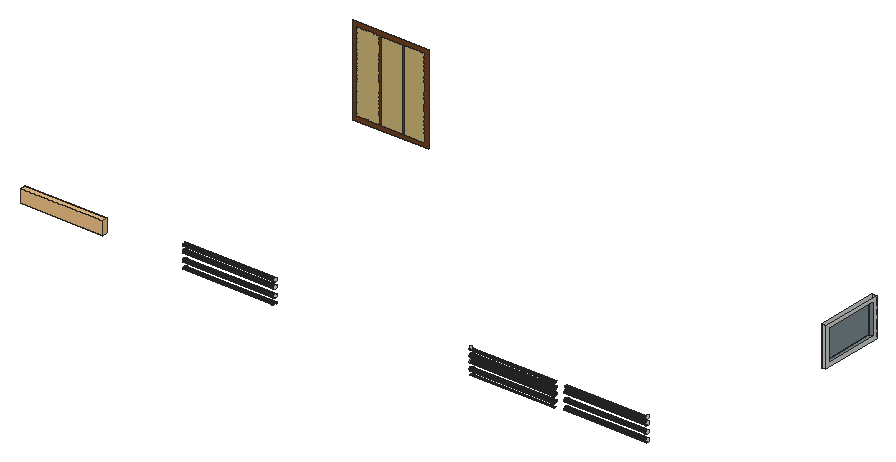
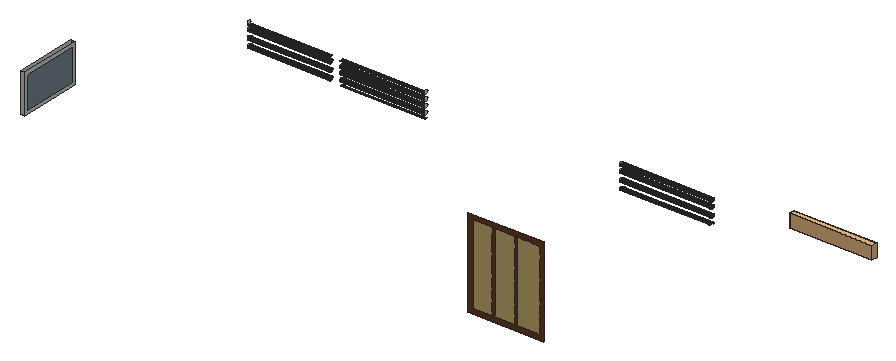
# SketchUp Ruby script. Lengths in inches.
U = 1.inch
M = Sketchup.active_model
def pt(a) = Geom::Point3d.new(a.map { |v| v * U })
def face(e, loops, mat)
  f = e.add_face(loops[0].map { |a| pt(a) })
  loops[1..].each { |l| e.add_face(l.map { |a| pt(a) }).erase! }
  f.material = f.back_material = mat if mat
  f
end
# faces: each face lists its corners as indices into pts; further lists are holes
def faces(e, pts, list, mat = nil) = list.each { |f| face(e, (f[0].is_a?(Array) ? f : [f]).map { |l| l.map { |i| pts[i] } }, mat) }
# xy, xz, yz: faces in a plane at the given z, y or x. An outline is a flat list of corners, or four numbers for a rectangle; further outlines are holes
def ring(l) = l.size == 4 ? [[l[0], l[1]], [l[2], l[1]], [l[2], l[3]], [l[0], l[3]]] : l.each_slice(2).to_a
def flat(e, list, mat, &to3) = list.each { |f| face(e, (f[0].is_a?(Array) ? f : [f]).map { |l| ring(l).map { |u, v| to3.(u, v) } }, mat) }
def xy(e, z, list, mat = nil) = flat(e, list, mat) { |x, y| [x, y, z] }
def xz(e, y, list, mat = nil) = flat(e, list, mat) { |x, z| [x, y, z] }
def yz(e, x, list, mat = nil) = flat(e, list, mat) { |y, z| [x, y, z] }
def lines(e, pts, list) = list.each { |a, b| e.add_line(pt(pts[a]), pt(pts[b])) }
# prism: a flat outline (further loops are holes) pulled along v
def prism(e, loops, v, mat = nil)
  f = face(e, loops, mat); d = Geom::Vector3d.new(v.map { |x| x * U })
  f.pushpull(f.normal.samedirection?(d) ? d.length : -d.length)
end
def box(e, o, s, mat = nil) = prism(e, [[o, [o[0] + s[0], o[1], o[2]], [o[0] + s[0], o[1] + s[1], o[2]], [o[0], o[1] + s[1], o[2]]]], [0, 0, s[2]], mat)
def at(x, y, z, deg = 0) = Geom::Transformation.translation(pt([x, y, z])) * Geom::Transformation.rotation(ORIGIN, Z_AXIS, deg.degrees)
def axes(o, x, y, z) = Geom::Transformation.new([*x, 0, *y, 0, *z, 0, *pt(o).to_a, 1])
def part(name) = M.definitions.add(name)
# library, detail: a bought-in or finely detailed component or shape, given as its bounding box
def library(name, o, s) = part(name).tap { |d| box(d.entities, o, s) }
def detail(e, o, s) = box(e.add_group.entities, o, s)
def put(e, d, t, mat = nil) = e.add_instance(d, t).tap { |i| i.material = mat if mat }
def group(e, t, mat = nil) = e.add_group.tap { |g| g.transformation = t; g.material = mat if mat }.entities
root = M.entities
M.materials.add("[Basic Tile]").color = [203, 206, 202]
M.materials.add("[Color M07]").color = [58, 58, 58]
M.materials.add("[Formica Speckled Grey]").color = [120, 135, 142]
M.materials.add("[Window Covering 02]").color = [199, 178, 115]
M.materials.add("[Wood Veneer 01]1").color = [109, 63, 33]
c1 = library("Housedekho",[1.1875,0,0],[76.76,10.33,12])
xy(root,109.0625,[[1639.03,679.86,1649.41,818.6]],"[Basic Tile]")
xy(root,117.18,[[1639.03,687.97,1649.41,810.49]],"[Formica Speckled Grey]")
xz(root,679.86,[[1639.03,109.0625,1649.41,194.8125]],"[Basic Tile]")
xz(root,687.97,[[1639.03,117.18,1649.41,186.7]],"[Formica Speckled Grey]")
xz(root,810.49,[[1639.03,117.18,1649.41,186.7]],"[Formica Speckled Grey]")
xz(root,818.6,[[1639.03,109.0625,1649.41,194.8125]],"[Basic Tile]")
xz(root,868.79,[[457.96,110.125,505.09,287.57],[513.29,110.125,556.28,287.57],[564.47,110.125,606.03,287.57]],"[Window Covering 02]")
xz(root,868.79,[[[448.22,100.38,615.78,297.32],[457.96,110.125,606.03,287.57]],[505.09,110.125,513.29,287.57],[556.28,110.125,564.47,287.57]],"[Wood Veneer 01]1")
yz(root,716.4,[[319.3,81.86,320.31,82,321.24,82.38,322.04,83,322.66,83.8,323.05,84.74,323.18,85.74,323.05,86.74,322.66,87.68,322.04,88.48,321.24,89.09,320.31,89.48,319.3,89.61,318.3,89.48,317.37,89.09,316.56,88.48,315.95,87.68,315.5625,86.74,315.43,85.74,315.5625,84.74,315.95,83.8,316.56,83,317.37,82.38,318.3,82],[319.3,99.55,320.31,99.68,321.24,100.07,322.04,100.6875,322.66,101.49,323.05,102.42,323.18,103.43,323.05,104.43,322.66,105.36,322.04,106.17,321.24,106.78,320.31,107.17,319.3,107.3,318.3,107.17,317.37,106.78,316.56,106.17,315.95,105.36,315.5625,104.43,315.43,103.43,315.5625,102.42,315.95,101.49,316.56,100.6875,317.37,100.07,318.3,99.68],[319.3,113.8,320.31,113.93,321.24,114.32,322.04,114.9375,322.66,115.74,323.05,116.67,323.18,117.68,323.05,118.68,322.66,119.61,322.04,120.42,321.24,121.03,320.31,121.42,319.3,121.55,318.3,121.42,317.37,121.03,316.56,120.42,315.95,119.61,315.5625,118.68,315.43,117.68,315.5625,116.67,315.95,115.74,316.56,114.9375,317.37,114.32,318.3,113.93]])
yz(root,1134.85,[[337.34,76.33,336.35,76.46,335.43,76.84,334.65,77.45,334.04,78.24,333.66,79.16,333.53,80.14,333.66,81.13,334.04,82.05,334.65,82.84,335.43,83.44,336.35,83.83,337.34,83.96,338.33,83.83,339.25,83.44,340.04,82.84,340.64,82.05,341.02,81.13,341.15,80.14,341.02,79.16,340.64,78.24,340.04,77.45,339.25,76.84,338.33,76.46],[337.34,90.83,336.35,90.96,335.43,91.34,334.65,91.95,334.04,92.74,333.66,93.66,333.53,94.64,333.66,95.63,334.04,96.55,334.65,97.34,335.43,97.94,336.35,98.33,337.34,98.46,338.33,98.33,339.25,97.94,340.04,97.34,340.64,96.55,341.02,95.63,341.15,94.64,341.02,93.66,340.64,92.74,340.04,91.95,339.25,91.34,338.33,90.96],[337.34,103.39,336.35,103.52,335.43,103.9,334.65,104.51,334.04,105.3,333.66,106.22,333.53,107.21,333.66,108.19,334.04,109.11,334.65,109.9,335.43,110.51,336.35,110.89,337.34,111.02,338.33,110.89,339.25,110.51,340.04,109.9,340.64,109.11,341.02,108.19,341.15,107.21,341.02,106.22,340.64,105.3,340.04,104.51,339.25,103.9,338.33,103.52],[337.34,117.89,336.35,118.02,335.43,118.4,334.65,119.01,334.04,119.8,333.66,120.72,333.53,121.71,333.66,122.69,334.04,123.61,334.65,124.4,335.43,125.01,336.35,125.39,337.34,125.52,338.33,125.39,339.25,125.01,340.04,124.4,340.64,123.61,341.02,122.69,341.15,121.71,341.02,120.72,340.64,119.8,340.04,119.01,339.25,118.4,338.33,118.02]])
yz(root,1527,[[337.76,71.29,338.75,71.42,339.67,71.8,340.46,72.4,341.0625,73.19,341.44,74.11,341.57,75.1,341.44,76.09,341.0625,77.01,340.46,77.79,339.67,78.4,338.75,78.78,337.76,78.91,336.77,78.78,335.85,78.4,335.06,77.79,334.46,77.01,334.08,76.09,333.95,75.1,334.08,74.11,334.46,73.19,335.06,72.4,335.85,71.8,336.77,71.42],[337.76,88.16,338.75,88.29,339.67,88.67,340.46,89.28,341.0625,90.07,341.44,90.99,341.57,91.97,341.44,92.96,341.0625,93.88,340.46,94.67,339.67,95.28,338.75,95.66,337.76,95.79,336.77,95.66,335.85,95.28,335.06,94.67,334.46,93.88,334.08,92.96,333.95,91.97,334.08,90.99,334.46,90.07,335.06,89.28,335.85,88.67,336.77,88.29],[337.76,104.79,338.75,104.92,339.67,105.3,340.46,105.9,341.0625,106.69,341.44,107.61,341.57,108.6,341.44,109.59,341.0625,110.51,340.46,111.29,339.67,111.9,338.75,112.28,337.76,112.41,336.77,112.28,335.85,111.9,335.06,111.29,334.46,110.51,334.08,109.59,333.95,108.6,334.08,107.61,334.46,106.69,335.06,105.9,335.85,105.3,336.77,104.92],[337.76,118.41,338.75,118.54,339.67,118.92,340.46,119.53,341.0625,120.32,341.44,121.24,341.57,122.22,341.44,123.21,341.0625,124.13,340.46,124.92,339.67,125.53,338.75,125.91,337.76,126.04,336.77,125.91,335.85,125.53,335.06,124.92,334.46,124.13,334.08,123.21,333.95,122.22,334.08,121.24,334.46,120.32,335.06,119.53,335.85,118.92,336.77,118.54]])
yz(root,1639.03,[[[679.86,109.0625,818.6,194.8125],[687.97,117.18,810.49,186.7]]],"[Basic Tile]")
yz(root,1639.03,[[687.97,117.18,810.49,186.7]],"[Formica Speckled Grey]")
yz(root,1649.41,[[[679.86,109.0625,818.6,194.8125],[687.97,117.18,810.49,186.7]]],"[Basic Tile]")
p = [[716.4,315.43,68.74],[716.4,315.5625,69.74],[513.6,315.5625,69.74],[513.6,315.43,68.74],[716.4,323.05,69.74],[716.4,323.18,68.74],
  [513.6,323.18,68.74],[513.6,323.05,69.74],[1134.85,336.35,69.14],[1134.85,335.43,68.76],[1322.28,335.43,68.76],[1322.28,336.35,69.14],
  [1134.85,339.25,68.76],[1134.85,338.33,69.14],[1322.28,338.33,69.14],[1322.28,339.25,68.76],[1134.85,337.34,69.27],[1322.28,337.34,69.27],
  [716.4,315.95,70.68],[513.6,315.95,70.68],[716.4,322.66,70.68],[513.6,322.66,70.68],[716.4,316.56,71.48],[513.6,316.56,71.48],
  [716.4,322.04,71.48],[513.6,322.04,71.48],[1527,337.76,71.29],[1527,336.77,71.42],[1344.86,336.77,71.42],[1344.86,337.76,71.29],
  [1527,338.75,71.42],[1344.86,338.75,71.42],[1527,335.85,71.8],[1344.86,335.85,71.8],[1527,339.67,71.8],[1344.86,339.67,71.8],
  [716.4,317.37,72.09],[513.6,317.37,72.09],[716.4,321.24,72.09],[513.6,321.24,72.09],[1527,335.06,72.4],[1344.86,335.06,72.4],
  [1527,340.46,72.4],[1344.86,340.46,72.4],[716.4,318.3,72.48],[513.6,318.3,72.48],[716.4,320.31,72.48],[513.6,320.31,72.48],
  [1527,334.46,73.19],[1344.86,334.46,73.19],[1527,341.0625,73.19],[1344.86,341.0625,73.19],[716.4,319.3,72.61],[513.6,319.3,72.61],
  [1527,334.08,74.11],[1344.86,334.08,74.11],[1527,341.44,74.11],[1344.86,341.44,74.11],[1527,333.95,75.1],[1344.86,333.95,75.1],
  [1527,341.57,75.1],[1344.86,341.57,75.1],[1527,334.08,76.09],[1344.86,334.08,76.09],[1527,341.44,76.09],[1344.86,341.44,76.09],
  [1527,334.46,77.01],[1344.86,334.46,77.01],[1527,341.0625,77.01],[1344.86,341.0625,77.01],[1134.85,336.35,76.46],[1134.85,337.34,76.33],
  [1322.28,337.34,76.33],[1322.28,336.35,76.46],[1134.85,338.33,76.46],[1322.28,338.33,76.46],[1134.85,335.43,76.84],[1322.28,335.43,76.84],
  [1134.85,339.25,76.84],[1322.28,339.25,76.84],[1134.85,334.65,77.45],[1322.28,334.65,77.45],[1134.85,340.04,77.45],[1322.28,340.04,77.45],
  [1527,335.06,77.79],[1344.86,335.06,77.79],[1527,340.46,77.79],[1344.86,340.46,77.79],[1134.85,334.04,78.24],[1322.28,334.04,78.24],
  [1134.85,340.64,78.24],[1322.28,340.64,78.24],[1527,335.85,78.4],[1344.86,335.85,78.4],[1527,339.67,78.4],[1344.86,339.67,78.4],
  [1134.85,333.66,79.16],[1322.28,333.66,79.16],[1134.85,341.02,79.16],[1322.28,341.02,79.16],[1527,336.77,78.78],[1344.86,336.77,78.78],
  [1527,338.75,78.78],[1344.86,338.75,78.78],[1527,337.76,78.91],[1344.86,337.76,78.91],[1134.85,333.53,80.14],[1322.28,333.53,80.14],
  [1134.85,341.15,80.14],[1322.28,341.15,80.14],[1134.85,333.66,81.13],[1322.28,333.66,81.13],[1134.85,341.02,81.13],[1322.28,341.02,81.13],
  [1134.85,334.04,82.05],[1322.28,334.04,82.05],[1134.85,340.64,82.05],[1322.28,340.64,82.05],[716.4,319.3,81.86],[716.4,318.3,82],
  [513.6,318.3,82],[513.6,319.3,81.86],[716.4,320.31,82],[513.6,320.31,82],[716.4,317.37,82.38],[513.6,317.37,82.38],
  [716.4,321.24,82.38],[513.6,321.24,82.38],[1134.85,334.65,82.84],[1322.28,334.65,82.84],[1134.85,340.04,82.84],[1322.28,340.04,82.84],
  [716.4,316.56,83],[513.6,316.56,83],[716.4,322.04,83],[513.6,322.04,83],[1134.85,335.43,83.44],[1322.28,335.43,83.44],
  [1134.85,339.25,83.44],[1322.28,339.25,83.44],[716.4,315.95,83.8],[513.6,315.95,83.8],[716.4,322.66,83.8],[513.6,322.66,83.8],
  [1134.85,336.35,83.83],[1322.28,336.35,83.83],[1134.85,338.33,83.83],[1322.28,338.33,83.83],[716.4,315.5625,84.74],[513.6,315.5625,84.74],
  [716.4,323.05,84.74],[513.6,323.05,84.74],[1134.85,337.34,83.96],[1322.28,337.34,83.96],[716.4,315.43,85.74],[513.6,315.43,85.74],
  [716.4,323.18,85.74],[513.6,323.18,85.74],[716.4,315.5625,86.74],[513.6,315.5625,86.74],[716.4,323.05,86.74],[513.6,323.05,86.74],
  [716.4,315.95,87.68],[513.6,315.95,87.68],[716.4,322.66,87.68],[513.6,322.66,87.68],[716.4,316.56,88.48],[513.6,316.56,88.48],
  [716.4,322.04,88.48],[513.6,322.04,88.48],[1527,337.76,88.16],[1527,336.77,88.29],[1344.86,336.77,88.29],[1344.86,337.76,88.16],
  [1527,338.75,88.29],[1344.86,338.75,88.29],[1527,335.85,88.67],[1344.86,335.85,88.67],[1527,339.67,88.67],[1344.86,339.67,88.67],
  [716.4,317.37,89.09],[513.6,317.37,89.09],[716.4,321.24,89.09],[513.6,321.24,89.09],[1527,335.06,89.28],[1344.86,335.06,89.28],
  [1527,340.46,89.28],[1344.86,340.46,89.28],[716.4,318.3,89.48],[513.6,318.3,89.48],[716.4,320.31,89.48],[513.6,320.31,89.48],
  [1527,334.46,90.07],[1344.86,334.46,90.07],[1527,341.0625,90.07],[1344.86,341.0625,90.07],[716.4,319.3,89.61],[513.6,319.3,89.61],
  [1527,334.08,90.99],[1344.86,334.08,90.99],[1527,341.44,90.99],[1344.86,341.44,90.99],[1134.85,336.35,90.96],[1134.85,337.34,90.83],
  [1322.28,337.34,90.83],[1322.28,336.35,90.96],[1134.85,338.33,90.96],[1322.28,338.33,90.96],[1527,333.95,91.97],[1344.86,333.95,91.97],
  [1134.85,335.43,91.34],[1322.28,335.43,91.34],[1134.85,339.25,91.34],[1322.28,339.25,91.34],[1527,341.57,91.97],[1344.86,341.57,91.97],
  [1134.85,334.65,91.95],[1322.28,334.65,91.95],[1134.85,340.04,91.95],[1322.28,340.04,91.95],[1134.85,334.04,92.74],[1322.28,334.04,92.74],
  [1134.85,340.64,92.74],[1322.28,340.64,92.74],[1527,334.08,92.96],[1344.86,334.08,92.96],[1527,341.44,92.96],[1344.86,341.44,92.96],
  [1134.85,333.66,93.66],[1322.28,333.66,93.66],[1134.85,341.02,93.66],[1322.28,341.02,93.66],[1527,334.46,93.88],[1344.86,334.46,93.88],
  [1527,341.0625,93.88],[1344.86,341.0625,93.88],[1134.85,333.53,94.64],[1322.28,333.53,94.64],[1134.85,341.15,94.64],[1322.28,341.15,94.64],
  [1527,335.06,94.67],[1344.86,335.06,94.67],[1527,340.46,94.67],[1344.86,340.46,94.67],[1134.85,333.66,95.63],[1322.28,333.66,95.63],
  [1134.85,341.02,95.63],[1322.28,341.02,95.63],[1527,335.85,95.28],[1344.86,335.85,95.28],[1527,339.67,95.28],[1344.86,339.67,95.28],
  [1527,336.77,95.66],[1344.86,336.77,95.66],[1527,338.75,95.66],[1344.86,338.75,95.66],[1134.85,334.04,96.55],[1322.28,334.04,96.55],
  [1134.85,340.64,96.55],[1322.28,340.64,96.55],[1527,337.76,95.79],[1344.86,337.76,95.79],[1134.85,334.65,97.34],[1322.28,334.65,97.34],
  [1134.85,340.04,97.34],[1322.28,340.04,97.34],[1134.85,335.43,97.94],[1322.28,335.43,97.94],[1134.85,339.25,97.94],[1322.28,339.25,97.94],
  [1134.85,336.35,98.33],[1322.28,336.35,98.33],[1134.85,338.33,98.33],[1322.28,338.33,98.33],[1134.85,337.34,98.46],[1322.28,337.34,98.46],
  [716.4,319.3,99.55],[716.4,318.3,99.68],[513.6,318.3,99.68],[513.6,319.3,99.55],[716.4,320.31,99.68],[513.6,320.31,99.68],
  [716.4,317.37,100.07],[513.6,317.37,100.07],[716.4,321.24,100.07],[513.6,321.24,100.07],[716.4,316.56,100.6875],[513.6,316.56,100.6875],
  [716.4,322.04,100.6875],[513.6,322.04,100.6875],[716.4,315.95,101.49],[513.6,315.95,101.49],[716.4,322.66,101.49],[513.6,322.66,101.49],
  [716.4,315.5625,102.42],[513.6,315.5625,102.42],[716.4,323.05,102.42],[513.6,323.05,102.42],[716.4,315.43,103.43],[513.6,315.43,103.43],
  [716.4,323.18,103.43],[513.6,323.18,103.43],[716.4,315.5625,104.43],[513.6,315.5625,104.43],[716.4,323.05,104.43],[513.6,323.05,104.43],
  [1134.85,336.35,103.52],[1134.85,337.34,103.39],[1322.28,337.34,103.39],[1322.28,336.35,103.52],[1134.85,338.33,103.52],[1322.28,338.33,103.52],
  [1134.85,335.43,103.9],[1322.28,335.43,103.9],[1134.85,339.25,103.9],[1322.28,339.25,103.9],[1134.85,334.65,104.51],[1322.28,334.65,104.51],
  [1134.85,340.04,104.51],[1322.28,340.04,104.51],[716.4,315.95,105.36],[513.6,315.95,105.36],[716.4,322.66,105.36],[513.6,322.66,105.36],
  [1134.85,334.04,105.3],[1322.28,334.04,105.3],[1134.85,340.64,105.3],[1322.28,340.64,105.3],[1527,337.76,104.79],[1527,336.77,104.92],
  [1344.86,336.77,104.92],[1344.86,337.76,104.79],[1527,338.75,104.92],[1344.86,338.75,104.92],[1527,335.85,105.3],[1344.86,335.85,105.3],
  [1527,339.67,105.3],[1344.86,339.67,105.3],[1134.85,333.66,106.22],[1322.28,333.66,106.22],[1527,335.06,105.9],[1344.86,335.06,105.9],
  [1527,340.46,105.9],[1344.86,340.46,105.9],[1134.85,341.02,106.22],[1322.28,341.02,106.22],[716.4,316.56,106.17],[513.6,316.56,106.17],
  [716.4,322.04,106.17],[513.6,322.04,106.17],[1527,334.46,106.69],[1344.86,334.46,106.69],[1527,341.0625,106.69],[1344.86,341.0625,106.69],
  [716.4,317.37,106.78],[513.6,317.37,106.78],[716.4,321.24,106.78],[513.6,321.24,106.78],[1134.85,333.53,107.21],[1322.28,333.53,107.21],
  [1134.85,341.15,107.21],[1322.28,341.15,107.21],[1527,334.08,107.61],[1344.86,334.08,107.61],[1527,341.44,107.61],[1344.86,341.44,107.61],
  [716.4,318.3,107.17],[513.6,318.3,107.17],[716.4,320.31,107.17],[513.6,320.31,107.17],[716.4,319.3,107.3],[513.6,319.3,107.3],
  [1134.85,333.66,108.19],[1322.28,333.66,108.19],[1134.85,341.02,108.19],[1322.28,341.02,108.19],[1527,333.95,108.6],[1344.86,333.95,108.6],
  [1527,341.57,108.6],[1344.86,341.57,108.6],[1134.85,334.04,109.11],[1322.28,334.04,109.11],[1134.85,340.64,109.11],[1322.28,340.64,109.11],
  [1527,334.08,109.59],[1344.86,334.08,109.59],[1527,341.44,109.59],[1344.86,341.44,109.59],[1134.85,334.65,109.9],[1322.28,334.65,109.9],
  [1134.85,340.04,109.9],[1322.28,340.04,109.9],[1527,334.46,110.51],[1344.86,334.46,110.51],[1527,341.0625,110.51],[1344.86,341.0625,110.51],
  [1134.85,335.43,110.51],[1322.28,335.43,110.51],[1134.85,339.25,110.51],[1322.28,339.25,110.51],[1527,335.06,111.29],[1344.86,335.06,111.29],
  [1134.85,336.35,110.89],[1322.28,336.35,110.89],[1134.85,338.33,110.89],[1322.28,338.33,110.89],[1527,340.46,111.29],[1344.86,340.46,111.29],
  [1134.85,337.34,111.02],[1322.28,337.34,111.02],[1527,335.85,111.9],[1344.86,335.85,111.9],[1527,339.67,111.9],[1344.86,339.67,111.9],
  [1527,336.77,112.28],[1344.86,336.77,112.28],[1527,338.75,112.28],[1344.86,338.75,112.28],[1527,337.76,112.41],[1344.86,337.76,112.41],
  [716.4,319.3,113.8],[716.4,318.3,113.93],[513.6,318.3,113.93],[513.6,319.3,113.8],[716.4,320.31,113.93],[513.6,320.31,113.93],
  [716.4,317.37,114.32],[513.6,317.37,114.32],[716.4,321.24,114.32],[513.6,321.24,114.32],[716.4,316.56,114.9375],[513.6,316.56,114.9375],
  [716.4,322.04,114.9375],[513.6,322.04,114.9375],[716.4,315.95,115.74],[513.6,315.95,115.74],[716.4,322.66,115.74],[513.6,322.66,115.74],
  [716.4,315.5625,116.67],[513.6,315.5625,116.67],[716.4,323.05,116.67],[513.6,323.05,116.67],[716.4,315.43,117.68],[513.6,315.43,117.68],
  [716.4,323.18,117.68],[513.6,323.18,117.68],[716.4,315.5625,118.68],[513.6,315.5625,118.68],[716.4,323.05,118.68],[513.6,323.05,118.68],
  [1134.85,336.35,118.02],[1134.85,337.34,117.89],[1322.28,337.34,117.89],[1322.28,336.35,118.02],[1134.85,338.33,118.02],[1322.28,338.33,118.02],
  [1134.85,335.43,118.4],[1322.28,335.43,118.4],[1134.85,339.25,118.4],[1322.28,339.25,118.4],[1134.85,334.65,119.01],[1322.28,334.65,119.01],
  [1527,337.76,118.41],[1527,336.77,118.54],[1344.86,336.77,118.54],[1344.86,337.76,118.41],[1527,338.75,118.54],[1344.86,338.75,118.54],
  [1134.85,340.04,119.01],[1322.28,340.04,119.01],[1527,335.85,118.92],[1344.86,335.85,118.92],[1527,339.67,118.92],[1344.86,339.67,118.92],
  [716.4,315.95,119.61],[513.6,315.95,119.61],[716.4,322.66,119.61],[513.6,322.66,119.61],[1527,335.06,119.53],[1344.86,335.06,119.53],
  [1527,340.46,119.53],[1344.86,340.46,119.53],[1134.85,334.04,119.8],[1322.28,334.04,119.8],[1134.85,340.64,119.8],[1322.28,340.64,119.8]]
faces(root,p,[[0,1,2,3],[4,5,6,7],[8,9,10,11],[12,13,14,15],[16,8,11,17],[13,16,17,14],[1,18,19,2],[20,4,7,21],
  [18,22,23,19],[24,20,21,25],[26,27,28,29],[30,26,29,31],[27,32,33,28],[34,30,31,35],[22,36,37,23],[38,24,25,39],
  [32,40,41,33],[42,34,35,43],[36,44,45,37],[46,38,39,47],[40,48,49,41],[50,42,43,51],[44,52,53,45],[52,46,47,53],
  [48,54,55,49],[56,50,51,57],[54,58,59,55],[60,56,57,61],[58,62,63,59],[64,60,61,65],[62,66,67,63],[68,64,65,69],
  [70,71,72,73],[71,74,75,72],[76,70,73,77],[74,78,79,75],[80,76,77,81],[78,82,83,79],[66,84,85,67],[86,68,69,87],
  [88,80,81,89],[82,90,91,83],[84,92,93,85],[94,86,87,95],[96,88,89,97],[90,98,99,91],[92,100,101,93],[102,94,95,103],
  [100,104,105,101],[104,102,103,105],[106,96,97,107],[98,108,109,99],[110,106,107,111],[108,112,113,109],[114,110,111,115],[112,116,117,113],
  [118,119,120,121],[122,118,121,123],[119,124,125,120],[126,122,123,127],[128,114,115,129],[116,130,131,117],[124,132,133,125],[134,126,127,135],
  [136,128,129,137],[130,138,139,131],[132,140,141,133],[142,134,135,143],[144,136,137,145],[138,146,147,139],[140,148,149,141],[150,142,143,151],
  [152,144,145,153],[146,152,153,147],[148,154,155,149],[156,150,151,157],[154,158,159,155],[160,156,157,161],[158,162,163,159],[164,160,161,165],
  [162,166,167,163],[168,164,165,169],[170,171,172,173],[174,170,173,175],[171,176,177,172],[178,174,175,179],[166,180,181,167],[182,168,169,183],
  [176,184,185,177],[186,178,179,187],[180,188,189,181],[190,182,183,191],[184,192,193,185],[194,186,187,195],[188,196,197,189],[196,190,191,197],
  [192,198,199,193],[200,194,195,201],[202,203,204,205],[203,206,207,204],[198,208,209,199],[210,202,205,211],[206,212,213,207],[214,200,201,215],
  [216,210,211,217],[212,218,219,213],[220,216,217,221],[218,222,223,219],[208,224,225,209],[226,214,215,227],[228,220,221,229],[222,230,231,223],
  [224,232,233,225],[234,226,227,235],[236,228,229,237],[230,238,239,231],[232,240,241,233],[242,234,235,243],[244,236,237,245],[238,246,247,239],
  [240,248,249,241],[250,242,243,251],[248,252,253,249],[254,250,251,255],[256,244,245,257],[246,258,259,247],[252,260,261,253],[260,254,255,261],
  [262,256,257,263],[258,264,265,259],[266,262,263,267],[264,268,269,265],[270,266,267,271],[268,272,273,269],[274,270,271,275],[272,274,275,273],
  [276,277,278,279],[280,276,279,281],[277,282,283,278],[284,280,281,285],[282,286,287,283],[288,284,285,289],[286,290,291,287],[292,288,289,293],
  [290,294,295,291],[296,292,293,297],[294,298,299,295],[300,296,297,301],[298,302,303,299],[304,300,301,305],[306,307,308,309],[307,310,311,308],
  [312,306,309,313],[310,314,315,311],[316,312,313,317],[314,318,319,315],[302,320,321,303],[322,304,305,323],[324,316,317,325],[318,326,327,319],
  [328,329,330,331],[332,328,331,333],[329,334,335,330],[336,332,333,337],[338,324,325,339],[334,340,341,335],[342,336,337,343],[326,344,345,327],
  [320,346,347,321],[348,322,323,349],[340,350,351,341],[352,342,343,353],[346,354,355,347],[356,348,349,357],[358,338,339,359],[344,360,361,345],
  [350,362,363,351],[364,352,353,365],[354,366,367,355],[368,356,357,369],[366,370,371,367],[370,368,369,371],[372,358,359,373],[360,374,375,361],
  [362,376,377,363],[378,364,365,379],[380,372,373,381],[374,382,383,375],[376,384,385,377],[386,378,379,387],[388,380,381,389],[382,390,391,383],
  [384,392,393,385],[394,386,387,395],[396,388,389,397],[390,398,399,391],[392,400,401,393],[402,396,397,403],[398,404,405,399],[406,394,395,407],
  [408,402,403,409],[404,408,409,405],[400,410,411,401],[412,406,407,413],[410,414,415,411],[416,412,413,417],[414,418,419,415],[418,416,417,419],
  [420,421,422,423],[424,420,423,425],[421,426,427,422],[428,424,425,429],[426,430,431,427],[432,428,429,433],[430,434,435,431],[436,432,433,437],
  [434,438,439,435],[440,436,437,441],[438,442,443,439],[444,440,441,445],[442,446,447,443],[448,444,445,449],[450,451,452,453],[451,454,455,452],
  [456,450,453,457],[454,458,459,455],[460,456,457,461],[462,463,464,465],[466,462,465,467],[458,468,469,459],[463,470,471,464],[472,466,467,473],
  [446,474,475,447],[476,448,449,477],[470,478,479,471],[480,472,473,481],[482,460,461,483],[468,484,485,469]],"[Color M07]")
put(root,c1,axes([180.81,289.93,100.87],[2.385,0,0],[0,0,2.82],[0,-1,0]),"[Color M07]")
